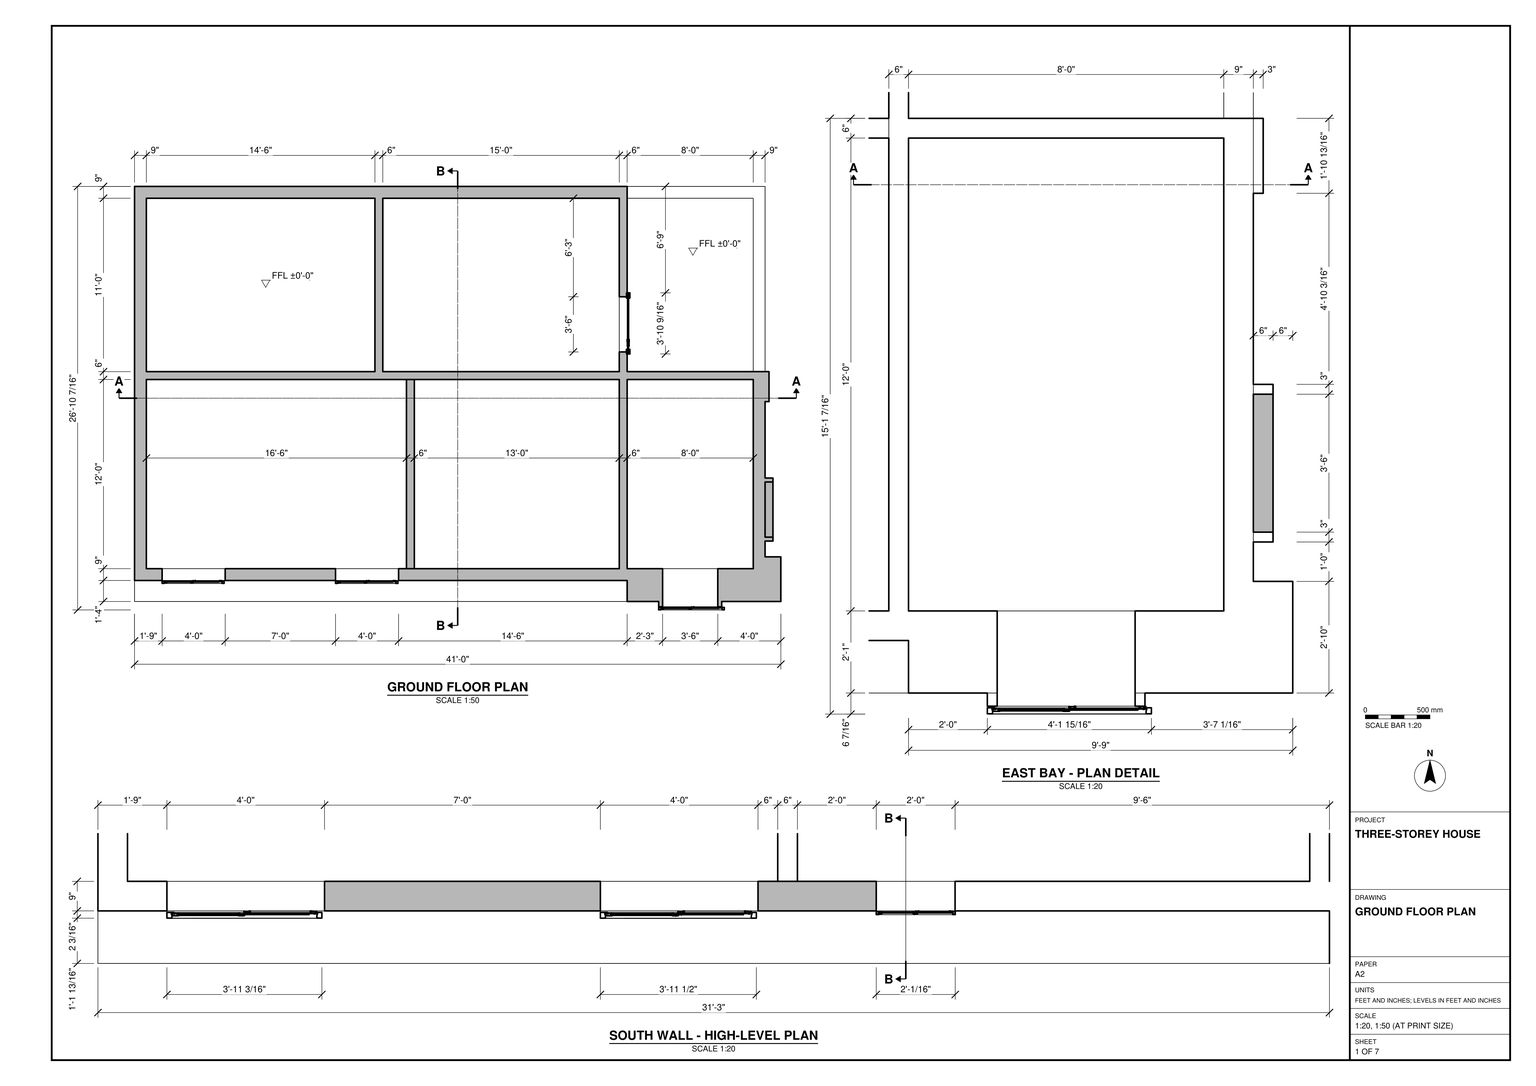
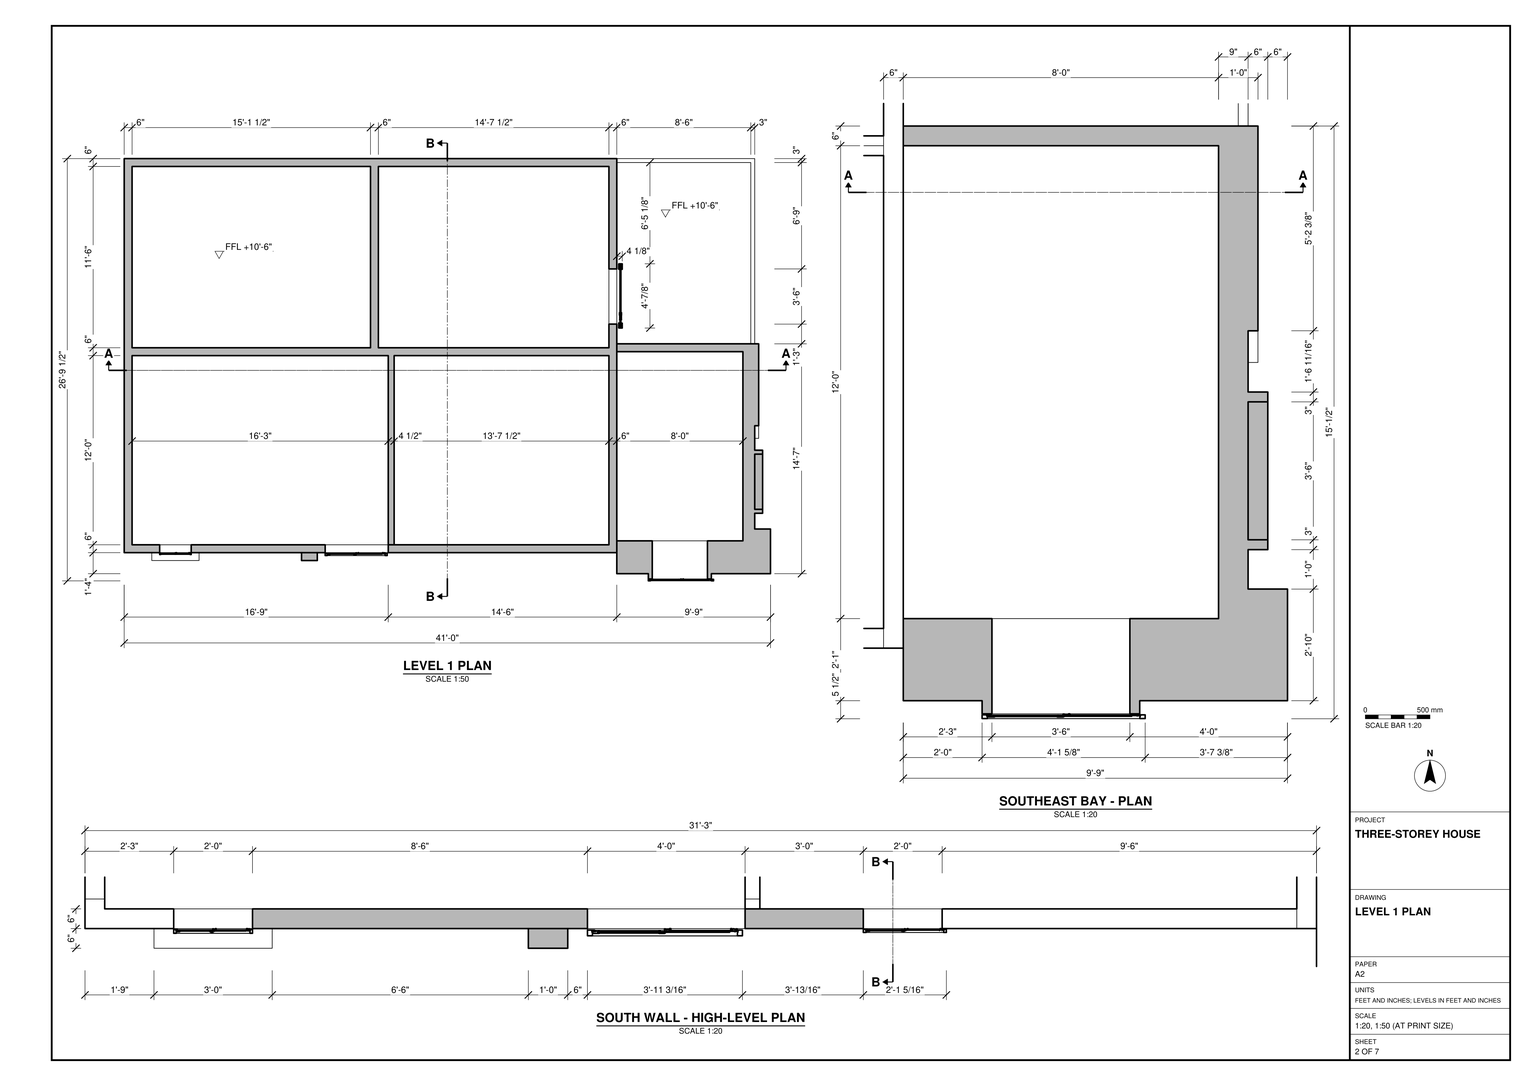
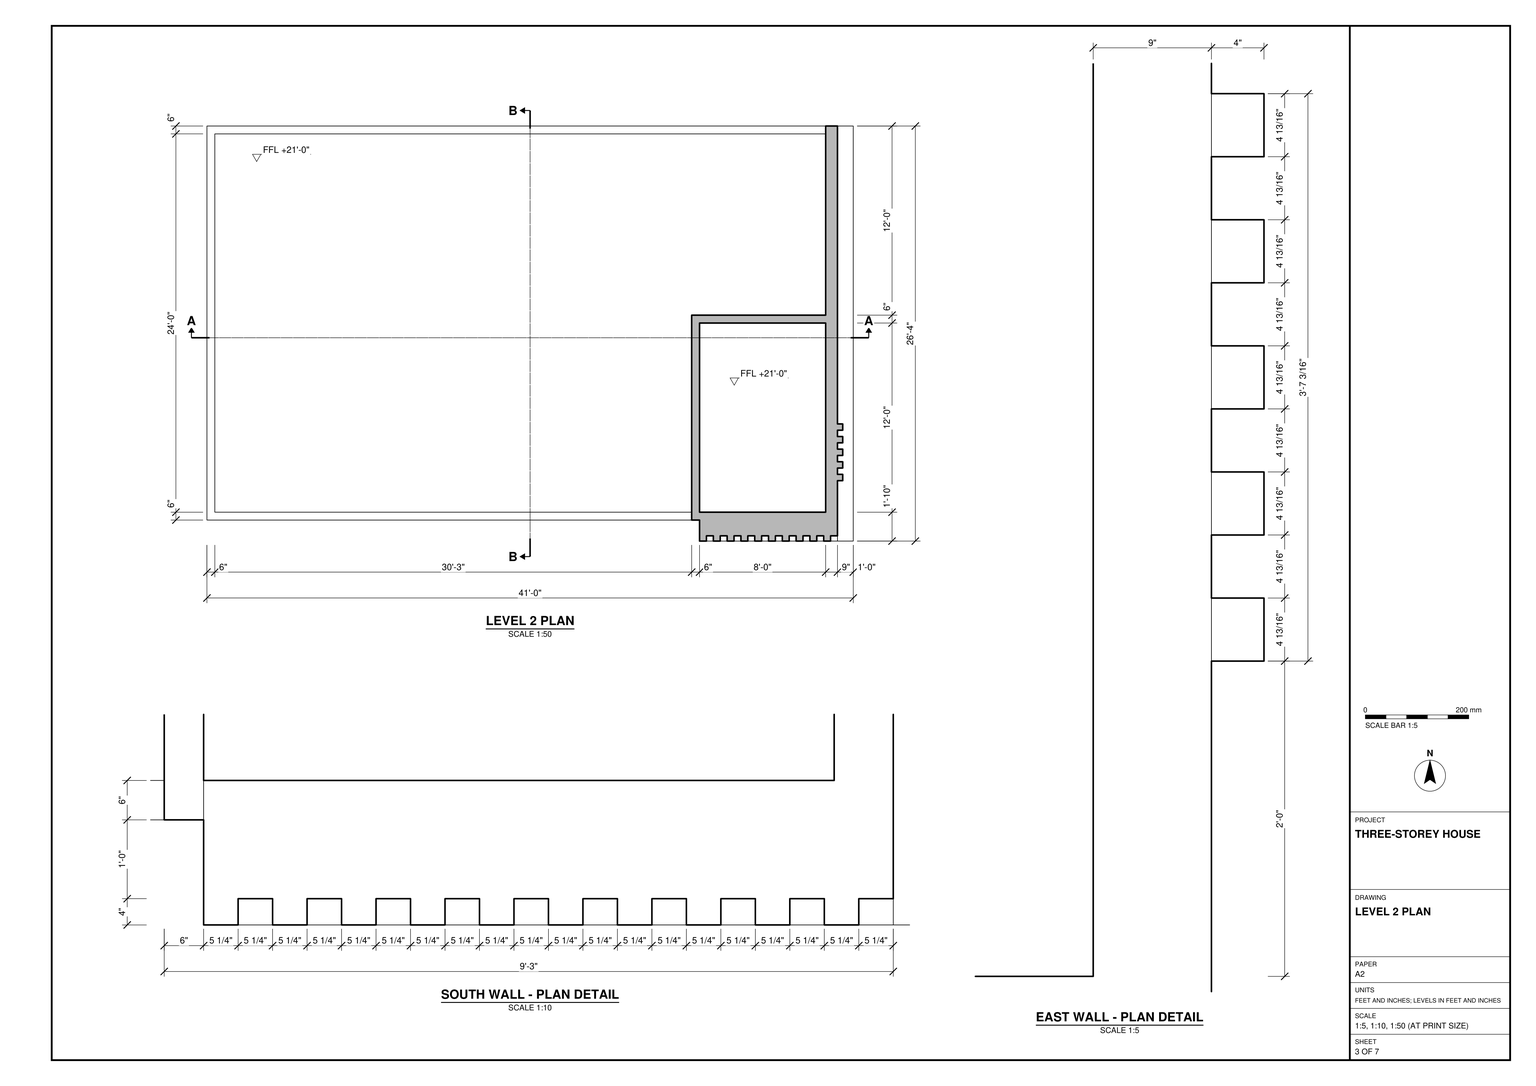
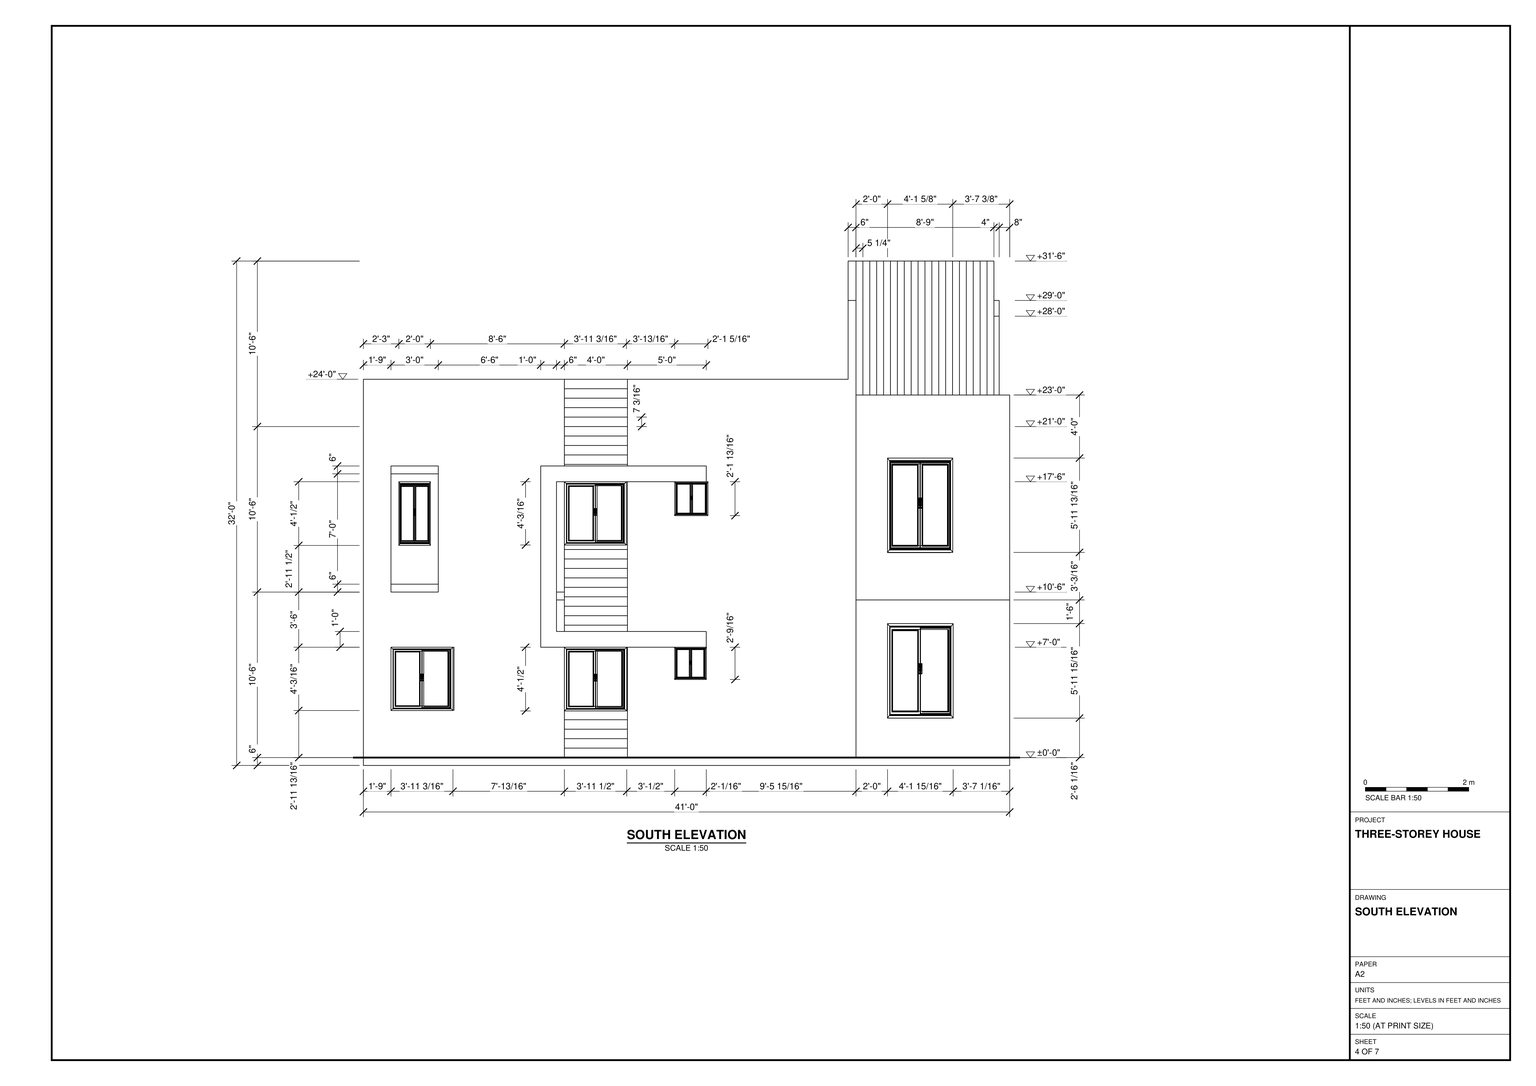
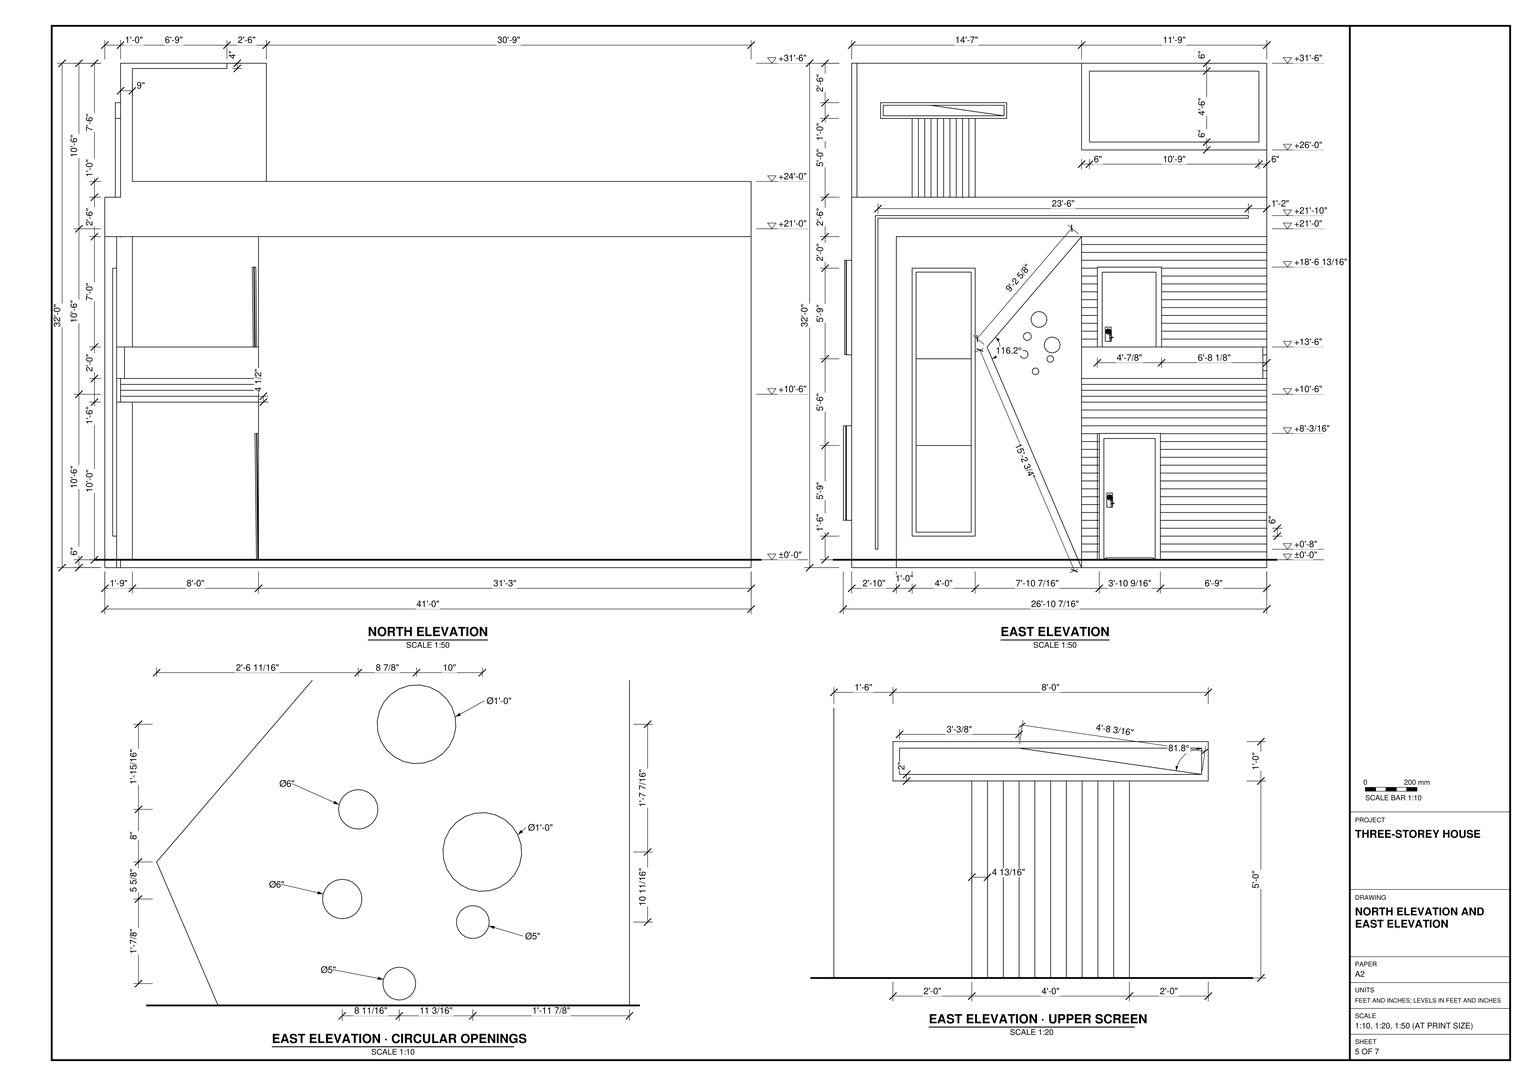
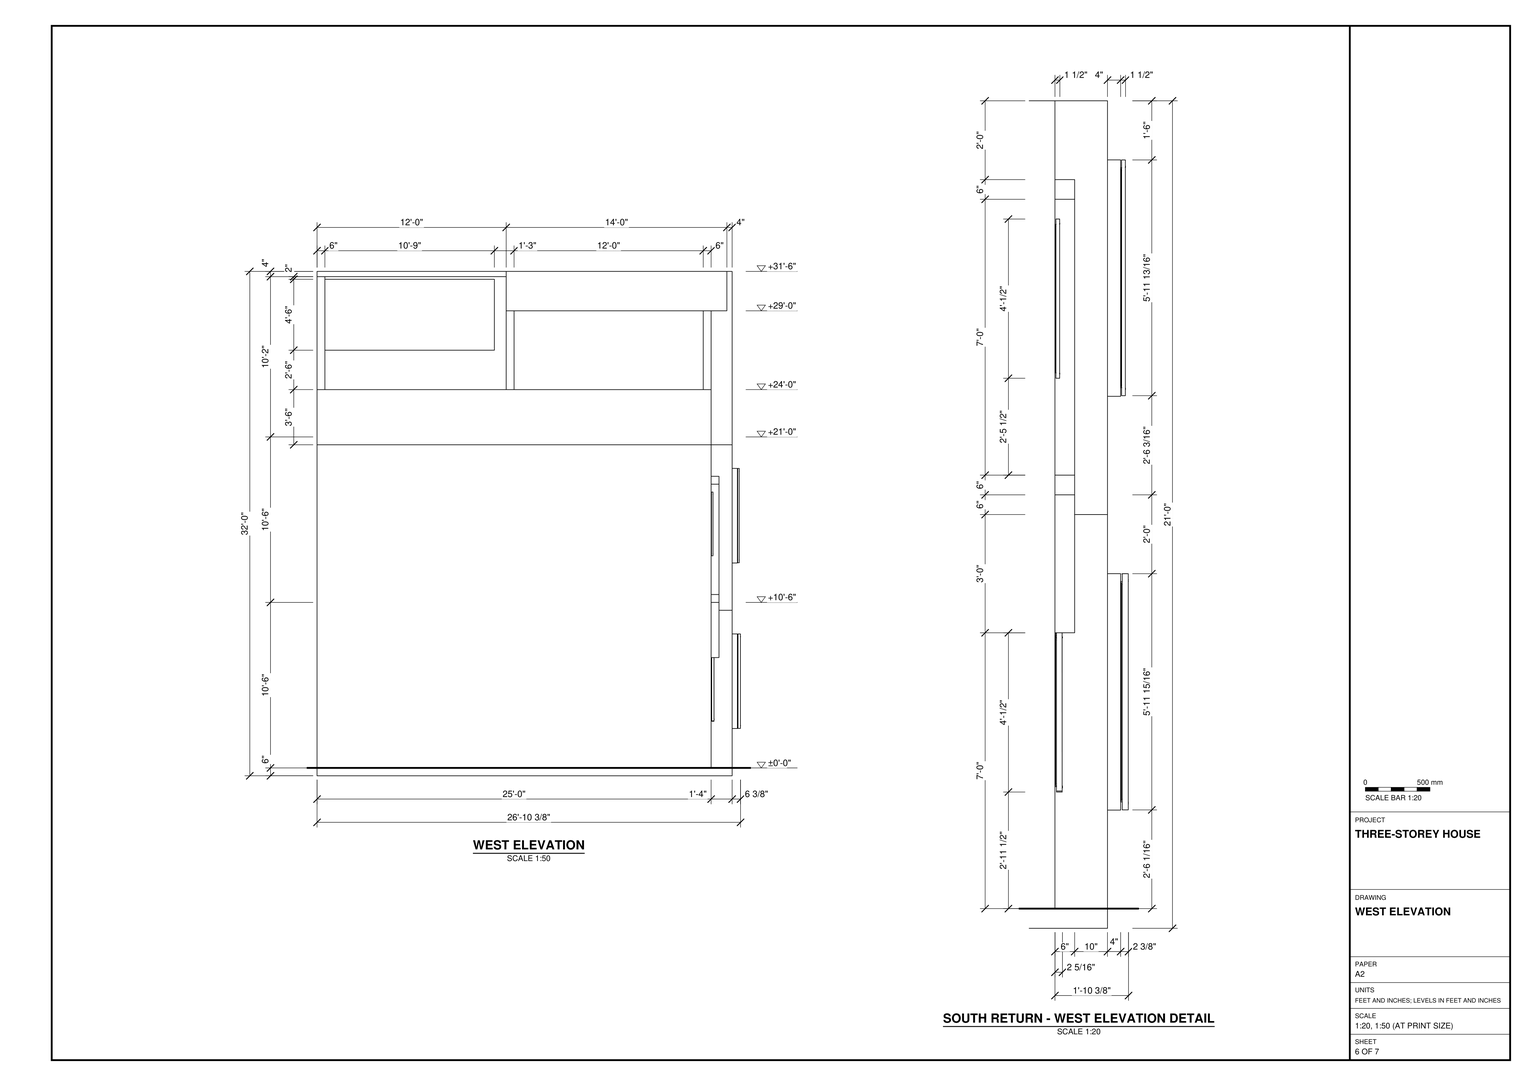
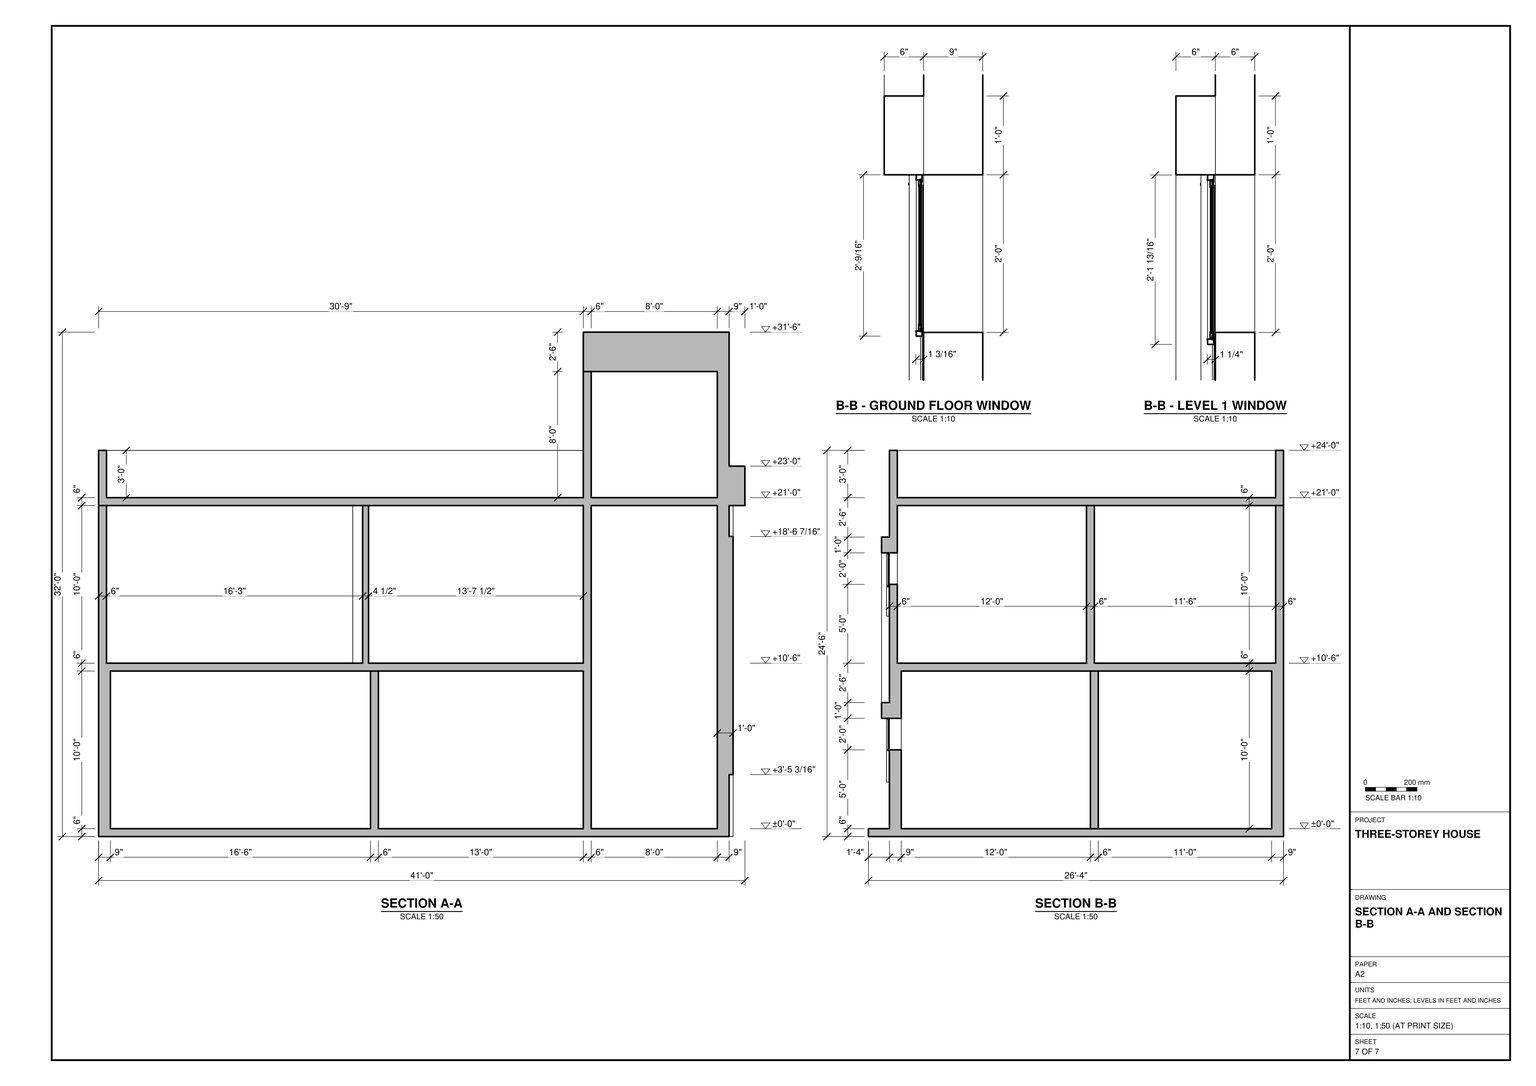
Build the three-storey house in SketchUp using task_files/diagram_01.pdf. Work in feet and inches. The overall extents are 41'-0" east to west, 26'-10 7/16" north to south and 32'-0" high. Set the finished floor levels at ±0'-0", +10'-6" and +21'-0".

Lay out the ground floor and first floor from their respective plans. The partitions change position and thickness between floors, so do not simply copy the ground floor upwards. Use the enlarged bay plans to shape the stepped southeast corner, including the reveals around its south-facing opening. Use the high-level plans as well as the floor plans to locate the openings along the south wall. At the top level, retain the broad open area beside the southeast enclosure. Follow the enlarged wall details for the repeated projections on the south face and the shorter run on the east face.

Model the slabs, roof, walls and opening units as drawn. Include stairs, built-in joinery and main furniture only where shown. Keep shell elements and individual furniture or joinery pieces in separate groups or components, and use components for repeated parts. Any decor or loose items shown may use suitable library components. Save one SketchUp model as output_files/three_storey_house_with_a_projecting_southeast_bay.skp.

# SketchUp Ruby script. Lengths in inches.
U = 1.inch
M = Sketchup.active_model
def pt(a) = Geom::Point3d.new(a.map { |v| v * U })
def face(e, loops, mat)
  f = e.add_face(loops[0].map { |a| pt(a) })
  loops[1..].each { |l| e.add_face(l.map { |a| pt(a) }).erase! }
  f.material = f.back_material = mat if mat
  f
end
# faces: each face lists its corners as indices into pts; further lists are holes
def faces(e, pts, list, mat = nil) = list.each { |f| face(e, (f[0].is_a?(Array) ? f : [f]).map { |l| l.map { |i| pts[i] } }, mat) }
# xy, xz, yz: faces in a plane at the given z, y or x. An outline is a flat list of corners, or four numbers for a rectangle; further outlines are holes
def ring(l) = l.size == 4 ? [[l[0], l[1]], [l[2], l[1]], [l[2], l[3]], [l[0], l[3]]] : l.each_slice(2).to_a
def flat(e, list, mat, &to3) = list.each { |f| face(e, (f[0].is_a?(Array) ? f : [f]).map { |l| ring(l).map { |u, v| to3.(u, v) } }, mat) }
def xy(e, z, list, mat = nil) = flat(e, list, mat) { |x, y| [x, y, z] }
def xz(e, y, list, mat = nil) = flat(e, list, mat) { |x, z| [x, y, z] }
def yz(e, x, list, mat = nil) = flat(e, list, mat) { |y, z| [x, y, z] }
def lines(e, pts, list) = list.each { |a, b| e.add_line(pt(pts[a]), pt(pts[b])) }
# prism: a flat outline (further loops are holes) pulled along v
def prism(e, loops, v, mat = nil)
  f = face(e, loops, mat); d = Geom::Vector3d.new(v.map { |x| x * U })
  f.pushpull(f.normal.samedirection?(d) ? d.length : -d.length)
end
def box(e, o, s, mat = nil) = prism(e, [[o, [o[0] + s[0], o[1], o[2]], [o[0] + s[0], o[1] + s[1], o[2]], [o[0], o[1] + s[1], o[2]]]], [0, 0, s[2]], mat)
def at(x, y, z, deg = 0) = Geom::Transformation.translation(pt([x, y, z])) * Geom::Transformation.rotation(ORIGIN, Z_AXIS, deg.degrees)
def axes(o, x, y, z) = Geom::Transformation.new([*x, 0, *y, 0, *z, 0, *pt(o).to_a, 1])
def part(name) = M.definitions.add(name)
# library, detail: a bought-in or finely detailed component or shape, given as its bounding box
def library(name, o, s) = part(name).tap { |d| box(d.entities, o, s) }
def detail(e, o, s) = box(e.add_group.entities, o, s)
def put(e, d, t, mat = nil) = e.add_instance(d, t).tap { |i| i.material = mat if mat }
def group(e, t, mat = nil) = e.add_group.tap { |g| g.transformation = t; g.material = mat if mat }.entities
root = M.entities
M.materials.add("C05_Golden_Blaze").color = [255, 123, 0]
M.materials.add("C06_Saffron_Kiss").color = [204, 102, 0]
M.materials.add("Denim_03_1K").color = [93, 106, 119]
M.materials.add("Glass_Basic_01").color = [0, 2, 119]
M.materials["Glass_Basic_01"].alpha = 0.25
M.materials.add("I01_Sky_Frost").color = [204, 204, 255]
M.materials.add("M05_Graphite_Haze").color = [114, 114, 114]
M.materials.add("M08_Obsidian_Black").color = [30, 30, 30]
M.materials.add("Plaster_03_1K").color = [121, 105, 83]
M.materials.add("Plaster_06_1K").color = [141, 135, 122]
M.materials.add("ThomThom - Waistcoat1").color = [155, 155, 155]
M.materials.add("ThomThom - Waistcoat2").color = [127, 127, 126]
c1 = library("porta+4",[0.2,-5.42,1.33],[46.55,4.72,83.21])
c2 = library("mesh-165",[-1596.32,-2661.67,-39.91],[1702.88,1739.15,82.5])
c3 = part("Group15")
put(c3.entities,c2,at(294.66,859.51,3.5))
g1 = group(root,at(0,20,0))
xy(g1,-6,[[0,-16,0,300,480,300,480,18,492,18,492,-16]])
xy(g1,0,[[0,-16,375,0],[9,9,207,153],[213,9,369,153],[375,9,471,153],[189,153,369,159],
  [9,159,183,291],[189,159,369,291],[375,159,471,291],[471,159,480,159,480,300,375,300,375,291,471,291]])
xy(g1,3,[[369,174,375,216]])
xy(g1,18,[[480,30,486,78]],"ThomThom - Waistcoat2")
xy(g1,21,[[480,33,486,75]],"ThomThom - Waistcoat2")
xy(g1,30,[[399,-20,447,-16]],"M08_Obsidian_Black")
xy(g1,33,[[402,-20,444,9]],"C06_Saffron_Kiss")
xy(g1,36,[[21.01,0,69.01,9],[153,0,201,9]])
xy(g1,60,[[237,0,261,9]])
xy(g1,84,[[21.01,0,69.01,9]])
xy(g1,84,[[135,-6,135,0,153,0,153,9,201,9,201,0,237,0,237,9,261,9,261,-6]],"M08_Obsidian_Black")
xy(g1,93,[[369,174,375,216]])
xy(g1,96,[[147,-6,261,0]],"M08_Obsidian_Black")
xy(g1,99,[[402,-20,444,9]],"C06_Saffron_Kiss")
xy(g1,102,[[399,-20,447,-16]],"M08_Obsidian_Black")
xy(g1,120,[[9,9,207,153],[207,9,213,153],[213,9,369,153],[9,153,183,159],[189,153,369,159],
  [9,159,183,291],[189,159,369,291],[375,159,480,300]])
xy(g1,126,[[6,6,201,150],[205.5,6,369,150],[6,156,187.5,294],[193.5,156,369,294],[375,159,477,297]])
xy(g1,126,[[21.01,-6,57.01,0]],"M08_Obsidian_Black")
xy(g1,129,[[369,174,375,216]])
xy(g1,132,[[21.01,-6,57.01,0]],"M08_Obsidian_Black")
xy(g1,138,[[477,159,480,159,480,300,375,300,375,297,477,297]])
xy(g1,156,[[399,-20,447,-16]],"M08_Obsidian_Black")
xy(g1,159,[[402,-20,444,9]],"C06_Saffron_Kiss")
xy(g1,162,[[27.01,0,51.01,6],[153,0,201,6]])
xy(g1,186,[[237,0,261,6]])
xy(g1,210,[[27.01,0,51.01,6]])
xy(g1,210,[[147,-6,147,0,153,0,153,6,201,6,201,0,237,0,237,6,261,6,261,-6]],"M08_Obsidian_Black")
xy(g1,216,[[21.01,-6,57.01,0]])
xy(g1,219,[[480,33,486,75],[369,174,375,216]])
xy(g1,222,[[21.01,-6,57.01,0],[135,-6,261,0]],"M08_Obsidian_Black")
xy(g1,222,[[480,30,486,78]],"ThomThom - Waistcoat2")
xy(g1,225,[[402,-20,444,9]],"C06_Saffron_Kiss")
xy(g1,228,[[399,-20,447,-16]],"M08_Obsidian_Black")
xy(g1,246,[[0,6,6,150],[6,6,201,150],[201,6,205.5,150],[205.5,6,369,150],[375,9,471,153],
  [0,150,187.5,156],[187.5,150,193.5,300],[193.5,150,369,156],[375,153,471,159],[0,156,6,159],
  [6,156,187.5,294],[193.5,156,369,294],[0,159,6,294],[375,159,471,300],[471,159,492,300],
  [0,294,187.5,300],[193.5,294,369,300]])
xy(g1,246,[[480,18,492,159]],"Denim_03_1K")
xy(g1,252,[[6,6,369,6,369,156,471,156,471,294,6,294],[375,6,471,150]])
xy(g1,276,[[380.25,-16,385.5,-12],[390.75,-16,396,-12],[401.25,-16,406.5,-12],[411.75,-16,417,-12],[422.25,-16,427.5,-12],
  [432.75,-16,438,-12],[443.25,-16,448.5,-12],[453.75,-16,459,-12],[464.25,-16,469.5,-12],[474.75,-16,480,-12],
  [480,-16,492,-16,492,300,480,300,480,73.2,484,73.2,484,68.4,480,68.4,480,63.6,484,63.6,484,58.8,480,58.8,480,54,484,54,484,49.2,480,49.2,480,44.4,484,44.4,484,39.6,480,39.6,480,34.8,484,34.8,484,30,480,30]],"Denim_03_1K")
xy(g1,288,[[0,0,369,0,369,6,6,6,6,294,471,294,471,300,0,300]])
xy(g1,318,[[471,165,480,294]])
xy(g1,336,[[480,6,484,30],[480,34.8,484,39.6],[480,44.4,484,49.2],[480,54,484,58.8],[480,63.6,484,68.4],
  [480,73.2,484,78],[480,78,484,102]],"Denim_03_1K")
xy(g1,338,[[480,8,484,30],[480,30,484,78],[480,78,484,100]],"Denim_03_1K")
xy(g1,346,[[480,8,484,100]],"Denim_03_1K")
xy(g1,348,[[369,-12,375,0],[369,6,375,150],[375,6,471,150]])
xy(g1,348,[[480,6,484,102]],"Denim_03_1K")
xy(g1,372,[[471,165,480,294]])
xy(g1,374,[[399,156,471,300]])
xy(g1,378,[[375,-16,380.25,-16,380.25,-12,385.5,-12,385.5,-16,390.75,-16,390.75,-12,396,-12,396,-16,401.25,-16,401.25,-12,406.5,-12,406.5,-16,411.75,-16,411.75,-12,417,-12,417,-16,422.25,-16,422.25,-12,427.5,-12,427.5,-16,432.75,-16,432.75,-12,438,-12,438,-16,443.25,-16,443.25,-12,448.5,-12,448.5,-16,453.75,-16,453.75,-12,459,-12,459,-16,464.25,-16,464.25,-12,469.5,-12,469.5,-16,474.75,-16,474.75,-12,480,-12,480,156,369,156,369,-12,375,-12],[399,156,480,300]])
xz(g1,-20,[[[399,30,447,102],[402,33,444,99]],[[399,156,447,228],[402,159,444,225]]],"M08_Obsidian_Black")
xz(g1,-16,[[[0,-6,492,-6,492,120,375,120,375,0,0,0],[399,30,447,102]],[[375,120,492,276],[399,156,447,228]],[375,276,380.25,378],[385.5,276,390.75,378],[396,276,401.25,378],
  [406.5,276,411.75,378],[417,276,422.25,378],[427.5,276,432.75,378],[438,276,443.25,378],[448.5,276,453.75,378],
  [459,276,464.25,378],[469.5,276,474.75,378]],"Denim_03_1K")
xz(g1,-12,[[369,348,375,378]])
xz(g1,-12,[[380.25,276,385.5,378],[390.75,276,396,378],[401.25,276,406.5,378],[411.75,276,417,378],[422.25,276,427.5,378],
  [432.75,276,438,378],[443.25,276,448.5,378],[453.75,276,459,378],[464.25,276,469.5,378],[474.75,276,480,378]],"Denim_03_1K")
xz(g1,-6,[[135,84,261,84,261,96,147,96,147,210,261,210,261,222,135,222],[21.01,126,57.01,132],[21.01,216,57.01,222]],"M08_Obsidian_Black")
xz(g1,0,[[[0,0,153,0,153,84,135,84,135,222,57.01,222,57.01,126,21.01,126,21.01,222,153,222,153,288,0,288],[21.01,36,69.01,84]],[201,0,375,0,375,348,369,348,369,288,201,288,201,222,261,222,261,186,237,186,237,210,201,210,201,96,261,96,261,60,237,60,237,84,201,84],[135,84,153,84,153,96,147,96,147,210,153,210,153,222,135,222],[153,86.4,201,93.6],[153,93.6,201,96],
  [147,96,153,120],[147,120,153,126],[147,126,153,210]])
xz(g1,0,[[153,0,201,7.2],[153,7.2,201,14.4],[153,14.4,201,21.6],[153,21.6,201,28.8],[153,28.8,201,36],
  [153,96,201,100.8],[153,100.8,201,108],[153,108,201,115.2],[153,115.2,201,122.4],[153,122.4,201,129.6],
  [153,129.6,201,136.8],[153,136.8,201,144],[153,144,201,151.2],[153,151.2,201,158.4],[153,158.4,201,162],
  [153,222,201,223.2],[153,223.2,201,230.4],[153,230.4,201,237.6],[153,237.6,201,244.8],[153,244.8,201,252],
  [153,252,201,259.2],[153,259.2,201,266.4],[153,266.4,201,273.6],[153,273.6,201,280.8],[153,280.8,201,288]],"C06_Saffron_Kiss")
xz(g1,0,[[[21.01,132,57.01,216],[27.01,162,51.01,210]]],"M08_Obsidian_Black")
xz(g1,6,[[[6,126,6,246,201,246,201,210,153,210,153,162,201,162,201,126],[27.01,162,51.01,210]],[[205.5,126,369,246],[237,186,261,210]],[201,162,205.5,210],[6,252,369,288],[375,252,471,348]])
xz(g1,6,[[480,336,484,348]],"Denim_03_1K")
xz(g1,8,[[480,338,484,346]],"Denim_03_1K")
xz(g1,9,[[[9,0,9,120,207,120,207,84,153,84,153,36,207,36,207,0],[21.01,36,69.01,84]],[[213,0,213,36,201,36,201,84,213,84,213,120,369,120,369,0],[237,60,261,84]],[207,0,213,36],[[375,0,471,246],[402,159,444,225],[402,33,444,99]],[207,36,213,84],
  [207,84,213,120]])
xz(g1,18,[[480,-6,492,246]],"Denim_03_1K")
xz(g1,30,[[480,276,484,336]],"Denim_03_1K")
xz(g1,30,[[480,18,486,222]],"ThomThom - Waistcoat2")
xz(g1,33,[[480,21,486,219]],"ThomThom - Waistcoat2")
xz(g1,34.8,[[480,276,484,336]],"Denim_03_1K")
xz(g1,39.6,[[480,276,484,336]],"Denim_03_1K")
xz(g1,44.4,[[480,276,484,336]],"Denim_03_1K")
xz(g1,49.2,[[480,276,484,336]],"Denim_03_1K")
xz(g1,54,[[480,276,484,336]],"Denim_03_1K")
xz(g1,58.8,[[480,276,484,336]],"Denim_03_1K")
xz(g1,63.6,[[480,276,484,336]],"Denim_03_1K")
xz(g1,68.4,[[480,276,484,336]],"Denim_03_1K")
xz(g1,73.2,[[480,276,484,336]],"Denim_03_1K")
xz(g1,75,[[480,21,486,219]],"ThomThom - Waistcoat2")
xz(g1,78,[[480,18,486,222]],"ThomThom - Waistcoat2")
xz(g1,100,[[480,338,484,346]],"Denim_03_1K")
xz(g1,102,[[480,336,484,348]])
xz(g1,150,[[6,126,193.5,246],[193.5,126,201,246],[205.5,126,369,246],[375,252,471,348]])
xz(g1,153,[[9,0,207,120],[207,0,213,120],[213,0,369,120],[375,0,471,246]])
xz(g1,156,[[6,126,187.5,246],[193.5,126,369,246],[369,252,369,378,399,378,399,374,471,374,471,252]])
xz(g1,159,[[9,0,183,120],[189,0,369,120],[375,0,471,120],[471,0,483,120],[375,120,471,126],
  [471,120,480,120,480,138,477,138,477,126,471,126],[375,126,471,246],[471,126,471,246,483,246,483,162,477,162,477,126],[477,138,483,162]])
xz(g1,159,[[480,-6,483,0],[480,120,483,138]],"M05_Graphite_Haze")
xz(g1,165,[[471,318,480,372]])
xz(g1,174,[[369,3,375,93],[369,129,375,219]])
xz(g1,216,[[369,3,375,93],[369,129,375,219]])
xz(g1,291,[[9,0,183,120],[189,0,369,120]])
xz(g1,294,[[6,126,187.5,246],[193.5,126,369,246],[6,252,471,288],[471,318,480,372]])
xz(g1,297,[[375,126,477,138]])
xz(g1,297,[[375,138,477,162]],"Glass_Basic_01")
xz(g1,300,[[0,-6,480,0],[0,0,375,246],[375,120,480,124.5],[375,124.5,480,129],[375,129,480,133.5],
  [375,133.5,480,138],[0,246,0,288,471,288,471,374,399,374,399,378,480,378,480,276,492,276,492,246]])
yz(g1,0,[[-16,-6,300,0],[0,0,300,246],[0,246,300,288]])
yz(g1,6,[[6,126,150,246],[156,126,294,246],[6,252,294,288]])
yz(g1,9,[[9,0,153,120],[159,0,291,120]])
yz(g1,21.01,[[0,36,9,84]])
yz(g1,21.01,[[-6,126,0,132],[-6,216,0,222]],"M08_Obsidian_Black")
yz(g1,27.01,[[0,162,6,210]])
yz(g1,51.01,[[0,162,6,210]])
yz(g1,57.01,[[-6,126,0,132],[-6,216,0,222]],"M08_Obsidian_Black")
yz(g1,69.01,[[0,36,9,84]])
yz(g1,135,[[-6,84,0,222]],"M08_Obsidian_Black")
yz(g1,147,[[-6,96,0,210]],"M08_Obsidian_Black")
yz(g1,153,[[0,36,9,84],[0,162,6,210]])
yz(g1,183,[[159,0,291,120]])
yz(g1,187.5,[[156,126,294,246]])
yz(g1,189,[[159,0,291,120]])
yz(g1,193.5,[[156,126,294,246]])
yz(g1,201,[[0,36,9,84],[6,126,150,246],[0,162,6,210]])
yz(g1,205.5,[[6,126,150,246]])
yz(g1,207,[[9,0,153,120]])
yz(g1,213,[[9,0,153,120]])
yz(g1,237,[[0,60,9,84],[0,186,6,210]])
yz(g1,261,[[0,60,9,84],[0,186,6,210]])
yz(g1,261,[[-6,84,0,96],[-6,210,0,222]],"M08_Obsidian_Black")
yz(g1,369,[[9,0,153,120],[[159,0,291,120],[174,3,216,93]],[6,126,9,246],[9,126,150,246],[156,126,159,246],
  [[159,126,294,246],[174,129,216,219]],[6,252,150,348],[150,252,156,348],[0,288,6,348],[-12,348,156,378]])
yz(g1,375,[[-16,0,0,120],[9,0,153,120],[171,0,219,0,219,6,216,6,216,3,174,3,174,6,171,6],[171,6,174,12],[216,6,219,12],
  [171,12,174,18],[216,12,219,18],[171,18,174,24],[216,18,219,24],[171,24,174,30],
  [216,24,219,30],[171,30,174,36],[216,30,219,36],[171,36,174,42],[216,36,219,42],
  [171,42,174,48],[216,42,219,48],[171,48,174,54],[216,48,219,54],[171,54,174,60],
  [216,54,219,60],[171,60,174,66],[216,60,219,66],[171,66,174,72],[216,66,219,72],
  [171,72,174,78],[216,72,219,78],[171,78,174,84],[216,78,219,84],[171,84,174,90],
  [216,84,219,90],[171,90,174,90,174,93,216,93,216,90,219,90,219,96,171,96],[-16,120,0,246],[0,120,9,246],[9,120,153,246],
  [153,120,159,246],[159,120,300,126],[171,126,219,126,219,132,216,132,216,129,174,129,174,132,171,132],[297,126,300,132],[171,132,174,138],
  [216,132,219,138],[297,132,300,138],[171,138,174,144],[216,138,219,144],[171,144,174,150],
  [216,144,219,150],[171,150,174,156],[216,150,219,156],[171,156,174,162],[216,156,219,162],
  [171,162,174,168],[216,162,219,168],[171,168,174,174],[216,168,219,174],[171,174,174,180],
  [216,174,219,180],[171,180,174,186],[216,180,219,186],[171,186,174,192],[216,186,219,192],
  [171,192,174,198],[216,192,219,198],[171,198,174,204],[216,198,219,204],[171,204,174,210],
  [216,204,219,210],[171,210,174,216],[216,210,219,216],[171,216,174,216,174,219,216,219,216,216,219,216,219,222,171,222],[6,252,150,348]])
yz(g1,375,[[-16,246,-16,378,-12,378,-12,348,0,348,0,246]],"Denim_03_1K")
yz(g1,375,[[159,126,171,132],[219,126,297,132],[159,132,171,138],[219,132,297,138],[159,138,171,144],
  [219,138,297,144],[297,138,300,144],[159,144,171,150],[219,144,297,150],[297,144,300,150],
  [159,150,171,156],[219,150,297,156],[297,150,300,156],[159,156,171,162],[219,156,297,162],
  [297,156,300,162],[159,162,171,168],[219,162,300,168],[159,168,171,174],[219,168,300,174],
  [159,174,171,180],[219,174,300,180],[159,180,171,186],[219,180,300,186],[159,186,171,192],
  [219,186,300,192],[159,192,171,198],[219,192,300,198],[159,198,171,204],[219,198,300,204],
  [159,204,171,210],[219,204,300,210],[159,210,171,216],[219,210,300,216],[159,216,171,222],
  [219,216,300,222],[159,222,300,228],[159,228,300,234],[159,234,300,240],[159,240,300,246]],"M05_Graphite_Haze")
yz(g1,375,[[159,0,171,6],[219,0,300,6],[159,6,171,12],[219,6,300,12],[159,12,171,18],
  [219,12,300,18],[159,18,171,24],[219,18,300,24],[159,24,171,30],[219,24,300,30],
  [159,30,171,36],[219,30,300,36],[159,36,171,42],[219,36,300,42],[159,42,171,48],
  [219,42,300,48],[159,48,171,54],[219,48,300,54],[159,54,171,60],[219,54,300,60],
  [159,60,171,66],[219,60,300,66],[159,66,171,72],[219,66,300,72],[159,72,171,78],
  [219,72,300,78],[159,78,171,84],[219,78,300,84],[159,84,171,90],[219,84,300,90],
  [159,90,171,96],[219,90,300,96],[159,96,300,102],[159,102,300,108],[159,108,300,114],
  [159,114,300,120]],"ThomThom - Waistcoat1")
yz(g1,380.25,[[-16,276,-12,378]],"Denim_03_1K")
yz(g1,385.5,[[-16,276,-12,378]],"Denim_03_1K")
yz(g1,390.75,[[-16,276,-12,378]],"Denim_03_1K")
yz(g1,396,[[-16,276,-12,378]],"Denim_03_1K")
yz(g1,399,[[156,374,300,378]])
yz(g1,399,[[-20,30,-16,102],[-20,156,-16,228]],"M08_Obsidian_Black")
yz(g1,401.25,[[-16,276,-12,378]],"Denim_03_1K")
yz(g1,402,[[-20,33,9,99],[-20,159,9,225]],"C06_Saffron_Kiss")
yz(g1,406.5,[[-16,276,-12,378]],"Denim_03_1K")
yz(g1,411.75,[[-16,276,-12,378]],"Denim_03_1K")
yz(g1,417,[[-16,276,-12,378]],"Denim_03_1K")
yz(g1,422.25,[[-16,276,-12,378]],"Denim_03_1K")
yz(g1,427.5,[[-16,276,-12,378]],"Denim_03_1K")
yz(g1,432.75,[[-16,276,-12,378]],"Denim_03_1K")
yz(g1,438,[[-16,276,-12,378]],"Denim_03_1K")
yz(g1,443.25,[[-16,276,-12,378]],"Denim_03_1K")
yz(g1,444,[[-20,33,9,99],[-20,159,9,225]],"C06_Saffron_Kiss")
yz(g1,447,[[-20,30,-16,102],[-20,156,-16,228]],"M08_Obsidian_Black")
yz(g1,448.5,[[-16,276,-12,378]],"Denim_03_1K")
yz(g1,453.75,[[-16,276,-12,378]],"Denim_03_1K")
yz(g1,459,[[-16,276,-12,378]],"Denim_03_1K")
yz(g1,464.25,[[-16,276,-12,378]],"Denim_03_1K")
yz(g1,469.5,[[-16,276,-12,378]],"Denim_03_1K")
yz(g1,471,[[9,0,153,246],[6,252,150,348],[156,252,156,374,294,374,294,372,165,372,165,318,294,318,294,252],[294,288,300,374]])
yz(g1,474.75,[[-16,276,-12,378]],"Denim_03_1K")
yz(g1,477,[[159,126,297,138]])
yz(g1,477,[[159,138,297,162]],"Glass_Basic_01")
yz(g1,480,[[159,120,300,124.5],[159,124.5,300,129],[159,129,300,133.5],[159,133.5,300,138],[-12,276,30,276,30,336,6,336,6,348,102,348,102,336,78,336,78,276,300,276,300,312,159,312,159,378,-12,378],
  [34.8,276,39.6,336],[44.4,276,49.2,336],[54,276,58.8,336],[63.6,276,68.4,336],[73.2,276,78,336],
  [[159,312,300,378],[165,318,294,372]],[8,338,100,338,44.37,346,8,346]])
yz(g1,480,[[100,338,100,346,44.37,346]],"C05_Golden_Blaze")
yz(g1,480,[[33,21,75,219]],"I01_Sky_Frost")
yz(g1,480,[[159,-6,300,0]],"Plaster_03_1K")
yz(g1,480,[[[18,-6,159,-6,87,162,159,246,18,246],[30,18,78,222]]],"Plaster_06_1K")
yz(g1,483,[[123.95,140.98,124.6,141.07,125.2,141.32,125.72,141.71,126.11,142.23,126.36,142.83,126.45,143.48,126.36,144.13,126.11,144.73,125.72,145.25,125.2,145.65,124.6,145.9,123.95,145.98,123.3,145.9,122.7,145.65,122.18,145.25,121.78,144.73,121.53,144.13,121.45,143.48,121.53,142.83,121.78,142.23,122.18,141.71,122.7,141.32,123.3,141.07],[135.21,150.35,135.86,150.45,136.45,150.72,136.96,151.13,137.35,151.66,137.58,152.27,137.65,152.92,137.54,153.5625,137.28,154.16,136.87,154.66,136.34,155.05,135.73,155.28,135.08,155.35,134.4375,155.25,133.84,154.98,133.33,154.57,132.95,154.04,132.72,153.43,132.65,152.78,132.75,152.14,133.02,151.54,133.43,151.04,133.96,150.65,134.57,150.42],[115.26,153.36,116.04,153.46,116.76,153.76,117.38,154.24,117.86,154.86,118.16,155.58,118.26,156.36,118.16,157.14,117.86,157.86,117.38,158.48,116.76,158.96,116.04,159.26,115.26,159.36,114.49,159.26,113.76,158.96,113.14,158.48,112.66,157.86,112.37,157.14,112.26,156.36,112.37,155.58,112.66,154.86,113.14,154.24,113.76,153.76,114.49,153.46],[136.15,157.54,137.71,157.63,139.2,158.12,140.51,158.98,141.55,160.15,142.26,161.55,142.57,163.08,142.48,164.65,141.99,166.13,141.13,167.44,139.96,168.49,138.5625,169.1875,137.03,169.51,135.47,169.42,133.98,168.93,132.67,168.07,131.63,166.9,130.92,165.5,130.61,163.96,130.7,162.4,131.1875,160.91,132.05,159.6,133.22,158.5625,134.62,157.86],[117.75,167.01,118.53,167.13,119.25,167.44,119.86,167.93,120.32,168.56,120.61,169.29,120.7,170.06,120.59,170.84,120.27,171.56,119.79,172.17,119.16,172.64,118.43,172.92,117.65,173.01,116.875,172.9,116.16,172.58,115.54,172.1,115.08,171.47,114.79,170.74,114.7,169.96,114.82,169.1875,115.13,168.47,115.62,167.86,116.25,167.39,116.97,167.1],
  [126.13,176.99,127.69,177.08,129.18,177.57,130.49,178.43,131.53,179.6,132.24,181,132.55,182.53,132.46,184.09,131.97,185.58,131.11,186.89,129.94,187.93,128.54,188.64,127.01,188.95,125.45,188.86,123.96,188.375,122.65,187.51,121.61,186.34,120.9,184.95,120.59,183.41,120.68,181.85,121.17,180.36,122.03,179.05,123.2,178.01,124.6,177.3]],"C05_Golden_Blaze")
yz(g1,483,[[[159,-6,159,246,87,162],[136.15,157.54,134.62,157.86,133.22,158.5625,132.05,159.6,131.1875,160.91,130.7,162.4,130.61,163.96,130.92,165.5,131.63,166.9,132.67,168.07,133.98,168.93,135.47,169.42,137.03,169.51,138.5625,169.1875,139.96,168.49,141.13,167.44,141.99,166.13,142.48,164.65,142.57,163.08,142.26,161.55,141.55,160.15,140.51,158.98,139.2,158.12,137.71,157.63],[126.13,176.99,124.6,177.3,123.2,178.01,122.03,179.05,121.17,180.36,120.68,181.85,120.59,183.41,120.9,184.95,121.61,186.34,122.65,187.51,123.96,188.375,125.45,188.86,127.01,188.95,128.54,188.64,129.94,187.93,131.11,186.89,131.97,185.58,132.46,184.09,132.55,182.53,132.24,181,131.53,179.6,130.49,178.43,129.18,177.57,127.69,177.08],[117.75,167.01,116.97,167.1,116.25,167.39,115.62,167.86,115.13,168.47,114.82,169.1875,114.7,169.96,114.79,170.74,115.08,171.47,115.54,172.1,116.16,172.58,116.875,172.9,117.65,173.01,118.43,172.92,119.16,172.64,119.79,172.17,120.27,171.56,120.59,170.84,120.7,170.06,120.61,169.29,120.32,168.56,119.86,167.93,119.25,167.44,118.53,167.13],[115.26,153.36,114.49,153.46,113.76,153.76,113.14,154.24,112.66,154.86,112.37,155.58,112.26,156.36,112.37,157.14,112.66,157.86,113.14,158.48,113.76,158.96,114.49,159.26,115.26,159.36,116.04,159.26,116.76,158.96,117.38,158.48,117.86,157.86,118.16,157.14,118.26,156.36,118.16,155.58,117.86,154.86,117.38,154.24,116.76,153.76,116.04,153.46],[135.21,150.35,134.57,150.42,133.96,150.65,133.43,151.04,133.02,151.54,132.75,152.14,132.65,152.78,132.72,153.43,132.95,154.04,133.33,154.57,133.84,154.98,134.4375,155.25,135.08,155.35,135.73,155.28,136.34,155.05,136.87,154.66,137.28,154.16,137.54,153.5625,137.65,152.92,137.58,152.27,137.35,151.66,136.96,151.13,136.45,150.72,135.86,150.45],[123.95,140.98,123.3,141.07,122.7,141.32,122.18,141.71,121.78,142.23,121.53,142.83,121.45,143.48,121.53,144.13,121.78,144.73,122.18,145.25,122.7,145.65,123.3,145.9,123.95,145.98,124.6,145.9,125.2,145.65,125.72,145.25,126.11,144.73,126.36,144.13,126.45,143.48,126.36,142.83,126.11,142.23,125.72,141.71,125.2,141.32,124.6,141.07]]],"M05_Graphite_Haze")
yz(g1,484,[[30,276,34.8,336],[39.6,276,44.4,336],[49.2,276,54,336],[58.8,276,63.6,336],[68.4,276,73.2,336],
  [[6,336,102,348],[8,338,100,346]]],"Denim_03_1K")
yz(g1,486,[[33,21,75,87],[33,87,75,153],[33,153,75,219]],"Glass_Basic_01")
yz(g1,486,[[[30,18,78,222],[33,21,75,219]]],"ThomThom - Waistcoat2")
yz(g1,492,[[2,8,4,8,4,260,286,260,286,262,2,262]])
yz(g1,492,[[[-16,-6,18,-6,18,246,300,246,300,276,-16,276],[2,8,2,262,286,262,286,260,4,260,4,8]]],"Denim_03_1K")
p = [[480,87,162],[480,159,-6],[483,159,-6],[483,87,162],[480,159,246],[483,159,246],
  [183,159,0],[183,153,0],[189,9,120],[189,0,120],[369,9,120],[369,0,120],
  [9,9,120],[0,9,120],[9,291,120],[9,300,120],[183,291,120],[183,300,120],
  [189,291,120],[189,300,120],[187.5,6,246],[187.5,0,246],[369,6,246],[369,0,246],
  [471,6,348],[480,6,348],[471,150,348],[471,156,348],[201,0,210],[201,0,216],
  [153,0,216],[201,0,222],[201,0,86.4],[201,0,84],[375,174,6],[375,216,6]]
faces(g1,p,[[0,1,2,3],[4,0,3,5]],"M05_Graphite_Haze")
lines(g1,p,[[6,7],[8,9],[10,11],[12,13],[14,15],[16,17],[18,19],[20,21],[22,23],[24,25],[26,27],[28,29],
  [30,29],[29,31],[32,33],[34,35]])
put(g1,c1,axes([372.25,172.25,-1.54],[0,1,0],[-1,0,0],[0,0,1.15649]))
put(g1,c1,axes([374.3,170.79,124.45],[0,1.0506,0],[-1,0,0],[0,0,1.16383]))
put(g1,c3,axes([57.07,-1.01,85.75],[0.02771,0,0],[0,0,0.02771],[0,-0.02771,0]))
put(g1,c3,axes([256.33,-0.54,210.9375],[0.01485,0,0],[0,0,0.01485],[0,-0.01485,0]))
put(g1,c3,axes([189.07,-1.01,211.75],[0.02771,0,0],[0,0,0.02771],[0,-0.02771,0]))
put(g1,c3,axes([189.3,-1.02,85.76],[0.02789,0,0],[0,0,0.02789],[0,-0.02789,0]))
put(g1,c3,axes([255.39,-0.51,84.89],[0.01413,0,0],[0,0,0.01413],[0,-0.01413,0]))
put(g1,c3,axes([45.35,-0.66,211.76],[0.01409,0,0],[0,0,0.02789],[0,-0.01811,0]))
put(g1,c3,axes([436.95,-20.66,230.6],[0.02916,0,0],[0,0,0.04129],[0,-0.01811,0]))
put(g1,c3,axes([437.1875,-21.07,104.61],[0.02934,0,0],[0,0,0.04137],[0,-0.02934,0]))
